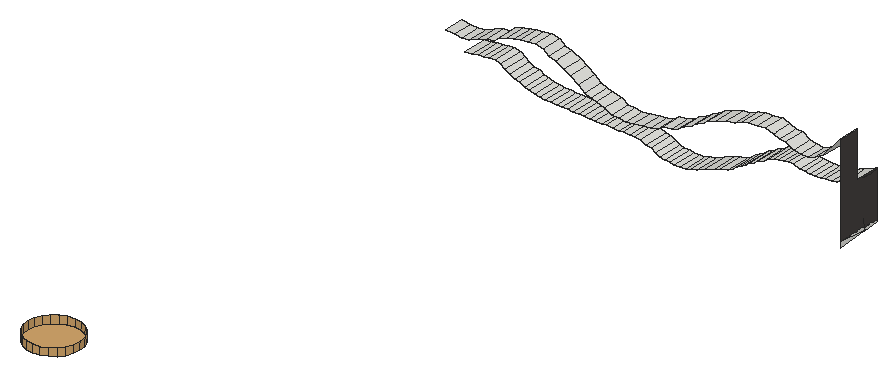
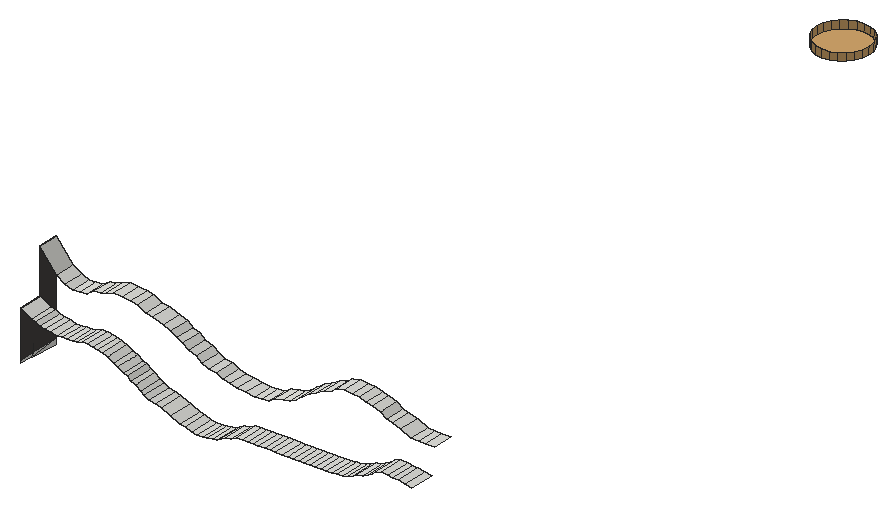
# SketchUp Ruby script. Lengths in inches.
U = 1.inch
M = Sketchup.active_model
def pt(a) = Geom::Point3d.new(a.map { |v| v * U })
def face(e, loops, mat)
  f = e.add_face(loops[0].map { |a| pt(a) })
  loops[1..].each { |l| e.add_face(l.map { |a| pt(a) }).erase! }
  f.material = f.back_material = mat if mat
  f
end
# faces: each face lists its corners as indices into pts; further lists are holes
def faces(e, pts, list, mat = nil) = list.each { |f| face(e, (f[0].is_a?(Array) ? f : [f]).map { |l| l.map { |i| pts[i] } }, mat) }
# xy, xz, yz: faces in a plane at the given z, y or x. An outline is a flat list of corners, or four numbers for a rectangle; further outlines are holes
def ring(l) = l.size == 4 ? [[l[0], l[1]], [l[2], l[1]], [l[2], l[3]], [l[0], l[3]]] : l.each_slice(2).to_a
def flat(e, list, mat, &to3) = list.each { |f| face(e, (f[0].is_a?(Array) ? f : [f]).map { |l| ring(l).map { |u, v| to3.(u, v) } }, mat) }
def xy(e, z, list, mat = nil) = flat(e, list, mat) { |x, y| [x, y, z] }
def xz(e, y, list, mat = nil) = flat(e, list, mat) { |x, z| [x, y, z] }
def yz(e, x, list, mat = nil) = flat(e, list, mat) { |y, z| [x, y, z] }
def lines(e, pts, list) = list.each { |a, b| e.add_line(pt(pts[a]), pt(pts[b])) }
# prism: a flat outline (further loops are holes) pulled along v
def prism(e, loops, v, mat = nil)
  f = face(e, loops, mat); d = Geom::Vector3d.new(v.map { |x| x * U })
  f.pushpull(f.normal.samedirection?(d) ? d.length : -d.length)
end
def box(e, o, s, mat = nil) = prism(e, [[o, [o[0] + s[0], o[1], o[2]], [o[0] + s[0], o[1] + s[1], o[2]], [o[0], o[1] + s[1], o[2]]]], [0, 0, s[2]], mat)
def at(x, y, z, deg = 0) = Geom::Transformation.translation(pt([x, y, z])) * Geom::Transformation.rotation(ORIGIN, Z_AXIS, deg.degrees)
def axes(o, x, y, z) = Geom::Transformation.new([*x, 0, *y, 0, *z, 0, *pt(o).to_a, 1])
def part(name) = M.definitions.add(name)
# library, detail: a bought-in or finely detailed component or shape, given as its bounding box
def library(name, o, s) = part(name).tap { |d| box(d.entities, o, s) }
def detail(e, o, s) = box(e.add_group.entities, o, s)
def put(e, d, t, mat = nil) = e.add_instance(d, t).tap { |i| i.material = mat if mat }
def group(e, t, mat = nil) = e.add_group.tap { |g| g.transformation = t; g.material = mat if mat }.entities
root = M.entities
M.materials.add("[Field Square Tile]").color = [211, 167, 108]
M.materials.add("[Granite Tile]1").color = [68, 65, 63]
xy(root,250.6875,[[2134.543,492.582,2133.831,492.675,2133.168,492.95,2132.598,493.387,2132.161,493.957,2131.886,494.62,2131.793,495.332,2131.886,496.043,2132.161,496.707,2132.598,497.276,2133.168,497.713,2133.831,497.988,2134.543,498.082,2135.254,497.988,2135.918,497.713,2136.487,497.276,2136.924,496.707,2137.199,496.043,2137.293,495.332,2137.199,494.62,2136.924,493.957,2136.487,493.387,2135.918,492.95,2135.254,492.675]],"[Field Square Tile]")
yz(root,2164.345,[[561.053,240.932,561.053,241.519,564.151,241.17],[564.185,241.167,564.151,241.17,564.184,241.173],[564.151,241.17,561.053,241.519,564.144,241.519,564.184,241.173],[564.184,241.173,564.144,241.519,565.74,241.519,565.74,241.293]])
yz(root,2164.345,[[561.053,241.519,561.053,251.165,563.178,251.165,563.178,246.426,565.74,246.426,565.74,241.519]],"[Granite Tile]1")
p = [[2144.767,563.178,241.17],[2144.767,565.74,241.17],[2145.237,565.74,241.121],[2145.237,563.178,241.121],[2145.843,565.74,241.09],[2145.843,563.178,241.09],
  [2146.41,565.74,241.138],[2146.41,563.178,241.138],[2147.05,565.74,241.346],[2147.05,563.178,241.346],[2143.769,563.178,241.332],[2143.769,565.74,241.332],
  [2144.237,565.74,241.243],[2144.237,563.178,241.243],[2143.35,563.178,241.566],[2143.35,565.74,241.566],[2147.641,565.74,241.456],[2147.641,563.178,241.456],
  [2148.576,565.74,241.847],[2148.576,563.178,241.847],[2142.844,563.178,241.837],[2142.844,565.74,241.837],[2142.271,563.178,241.967],[2142.271,565.74,241.967],
  [2149.581,565.74,242.229],[2149.581,563.178,242.229],[2141.69,563.178,242.199],[2141.69,565.74,242.199],[2141.064,563.178,242.277],[2141.064,565.74,242.277],
  [2150.142,565.74,242.424],[2150.142,563.178,242.424],[2135.217,563.178,242.35],[2135.217,565.74,242.35],[2135.799,565.74,242.342],[2135.799,563.178,242.342],
  [2136.381,565.74,242.334],[2136.381,563.178,242.334],[2136.963,565.74,242.326],[2136.963,563.178,242.326],[2137.683,565.74,242.317],[2137.683,563.178,242.317],
  [2138.153,565.74,242.312],[2138.153,563.178,242.312],[2138.794,565.74,242.304],[2138.794,563.178,242.304],[2139.458,565.74,242.296],[2139.458,563.178,242.296],
  [2139.91,565.74,242.291],[2139.91,563.178,242.291],[2140.548,565.74,242.283],[2140.548,563.178,242.283],[2131.735,563.178,242.466],[2131.735,565.74,242.466],
  [2132.311,565.74,242.428],[2132.311,563.178,242.428],[2132.89,565.74,242.403],[2132.89,563.178,242.403],[2133.47,565.74,242.385],[2133.47,563.178,242.385],
  [2134.052,565.74,242.371],[2134.052,563.178,242.371],[2134.634,565.74,242.36],[2134.634,563.178,242.36],[2150.86,565.74,242.605],[2150.86,563.178,242.605],
  [2130.607,563.178,242.599],[2130.607,565.74,242.599],[2131.167,565.74,242.518],[2131.167,563.178,242.518],[2130.054,563.178,242.75],[2130.054,565.74,242.75],
  [2151.373,565.74,242.907],[2151.373,563.178,242.907],[2129.566,563.178,242.921],[2129.566,565.74,242.921],[2129.075,563.178,243.216],[2129.075,565.74,243.216],
  [2151.745,565.74,243.144],[2151.745,563.178,243.144],[2152.294,565.74,243.516],[2152.294,563.178,243.516],[2128.527,563.178,243.332],[2128.527,565.74,243.332],
  [2127.982,563.178,243.589],[2127.982,565.74,243.589],[2152.768,565.74,243.711],[2152.768,563.178,243.711],[2127.501,563.178,243.88],[2127.501,565.74,243.88],
  [2153.099,565.74,244.02],[2153.099,563.178,244.02],[2127.124,563.178,244.194],[2127.124,565.74,244.194],[2123.336,563.178,243.992],[2123.336,565.74,243.992],
  [2124.039,565.74,244.076],[2124.039,563.178,244.076],[2153.543,565.74,244.206],[2153.543,563.178,244.206],[2124.738,565.74,244.207],[2124.738,563.178,244.207],
  [2125.323,565.74,244.266],[2125.323,563.178,244.266],[2126.527,563.178,244.387],[2126.527,565.74,244.387],[2154.132,565.74,244.569],[2154.132,563.178,244.569],
  [2125.864,565.74,244.296],[2125.864,563.178,244.296],[2154.602,565.74,244.757],[2154.602,563.178,244.757],[2155.219,565.74,245.125],[2155.219,563.178,245.125],
  [2140.415,561.053,245.064],[2140.415,563.178,245.064],[2141.125,563.178,244.949],[2141.125,561.053,244.949],[2141.839,563.178,244.867],[2141.839,561.053,244.867],
  [2142.745,563.178,245.007],[2142.745,561.053,245.007],[2143.689,563.178,245.121],[2143.689,561.053,245.121],[2139.702,561.053,245.459],[2139.702,563.178,245.459],
  [2144.454,563.178,245.254],[2144.454,561.053,245.254],[2155.723,565.74,245.32],[2155.723,563.178,245.32],[2159.424,563.178,245.272],[2159.424,565.74,245.272],
  [2159.982,565.74,245.235],[2159.982,563.178,245.235],[2160.536,565.74,245.216],[2160.536,563.178,245.216],[2161.101,565.74,245.34],[2161.101,563.178,245.34],
  [2145.206,563.178,245.41],[2145.206,561.053,245.41],[2156.205,565.74,245.411],[2156.205,563.178,245.411],[2157.771,563.178,245.552],[2157.771,565.74,245.552],
  [2158.379,565.74,245.346],[2158.379,563.178,245.346],[2158.873,565.74,245.309],[2158.873,563.178,245.309],[2161.733,565.74,245.423],[2161.733,563.178,245.423],
  [2145.84,563.178,245.775],[2145.84,561.053,245.775],[2156.753,565.74,245.481],[2156.753,563.178,245.481],[2162.311,565.74,245.516],[2162.311,563.178,245.516],
  [2138.827,561.053,245.671],[2138.827,563.178,245.671],[2157.235,565.74,245.59],[2157.235,563.178,245.59],[2162.691,565.74,245.763],[2162.691,563.178,245.763],
  [2138.152,561.053,245.834],[2138.152,563.178,245.834],[2137.564,561.053,246.129],[2137.564,563.178,246.129],[2146.636,563.178,245.88],[2146.636,561.053,245.88],
  [2163.16,565.74,245.896],[2163.16,563.178,245.896],[2147.349,563.178,246.16],[2147.349,561.053,246.16],[2164.345,565.74,246.426],[2164.345,563.178,246.426],
  [2136.933,561.053,246.633],[2136.933,563.178,246.633],[2147.946,563.178,246.573],[2147.946,561.053,246.573],[2136.119,561.053,247.185],[2136.119,563.178,247.185],
  [2148.736,563.178,246.902],[2148.736,561.053,246.902],[2123.942,561.053,246.79],[2123.942,563.178,246.79],[2124.721,563.178,246.747],[2124.721,561.053,246.747],
  [2125.468,563.178,246.831],[2125.468,561.053,246.831],[2122.988,561.053,246.838],[2122.988,563.178,246.838],[2126.51,563.178,247.251],[2126.51,561.053,247.251],
  [2149.338,563.178,247.347],[2149.338,561.053,247.347],[2135.407,561.053,247.553],[2135.407,563.178,247.553],[2127.384,563.178,247.546],[2127.384,561.053,247.546],
  [2150.012,563.178,247.615],[2150.012,561.053,247.615],[2128.046,563.178,247.657],[2128.046,561.053,247.657],[2134.516,561.053,248.059],[2134.516,563.178,248.059],
  [2150.599,563.178,248.057],[2150.599,561.053,248.057],[2128.679,563.178,248.162],[2128.679,561.053,248.162],[2133.825,561.053,248.257],[2133.825,563.178,248.257],
  [2151.364,563.178,248.322],[2151.364,561.053,248.322],[2129.473,563.178,248.408],[2129.473,561.053,248.408],[2160.161,561.053,248.295],[2160.161,563.178,248.295],
  [2160.87,563.178,248.218],[2160.87,561.053,248.218],[2161.687,563.178,248.558],[2161.687,561.053,248.558],[2133.294,561.053,248.687],[2133.294,563.178,248.687],
  [2152.475,563.178,248.655],[2152.475,561.053,248.655],[2159.45,561.053,248.42],[2159.45,563.178,248.42],[2130.172,563.178,248.521],[2130.172,561.053,248.521],
  [2158.653,561.053,248.895],[2158.653,563.178,248.895],[2130.866,563.178,248.723],[2130.866,561.053,248.723],[2162.622,563.178,249.022],[2162.622,561.053,249.022],
  [2131.565,563.178,248.801],[2131.565,561.053,248.801],[2132.462,561.053,248.851],[2132.462,563.178,248.851],[2153.248,563.178,248.795],[2153.248,561.053,248.795],
  [2154.111,563.178,249.194],[2154.111,561.053,249.194],[2157.949,561.053,248.962],[2157.949,563.178,248.962],[2157.31,561.053,249.206],[2157.31,563.178,249.206],
  [2164.345,563.178,251.165],[2164.345,561.053,251.165],[2154.784,563.178,249.323],[2154.784,561.053,249.323],[2156.565,561.053,249.478],[2156.565,563.178,249.478],
  [2155.707,563.178,249.406],[2155.707,561.053,249.406],[2134.543,492.582,251.5],[2133.831,492.675,251.5],[2133.831,492.675,250.6875],[2134.543,492.582,250.6875],
  [2135.254,492.675,251.5],[2135.254,492.675,250.6875],[2133.168,492.95,251.5],[2133.168,492.95,250.6875],[2135.918,492.95,251.5],[2135.918,492.95,250.6875],
  [2132.598,493.387,251.5],[2132.598,493.387,250.6875],[2136.487,493.387,251.5],[2136.487,493.387,250.6875],[2132.161,493.957,251.5],[2132.161,493.957,250.6875],
  [2136.924,493.957,251.5],[2136.924,493.957,250.6875],[2131.886,494.62,251.5],[2131.886,494.62,250.6875],[2137.199,494.62,251.5],[2137.199,494.62,250.6875],
  [2131.793,495.332,251.5],[2131.793,495.332,250.6875],[2137.293,495.332,251.5],[2137.293,495.332,250.6875],[2131.886,496.043,251.5],[2131.886,496.043,250.6875],
  [2137.199,496.043,251.5],[2137.199,496.043,250.6875],[2132.161,496.707,251.5],[2132.161,496.707,250.6875],[2136.924,496.707,251.5],[2136.924,496.707,250.6875],
  [2132.598,497.276,251.5],[2132.598,497.276,250.6875],[2136.487,497.276,251.5],[2136.487,497.276,250.6875],[2133.168,497.713,251.5],[2133.168,497.713,250.6875],
  [2135.918,497.713,251.5],[2135.918,497.713,250.6875],[2133.831,497.988,251.5],[2133.831,497.988,250.6875],[2135.254,497.988,251.5],[2135.254,497.988,250.6875],
  [2134.543,498.082,251.5],[2134.543,498.082,250.6875],[2164.345,564.963,246.171],[2164.345,563.948,246.265],[2164.345,564.144,241.519],[2164.345,564.042,242.384],
  [2164.345,565.74,246.273]]
faces(root,p,[[0,1,2,3],[3,2,4,5],[5,4,6,7],[7,6,8,9],[10,11,12,13],[13,12,1,0],[14,15,11,10],[9,8,16,17],
  [17,16,18,19],[20,21,15,14],[22,23,21,20],[19,18,24,25],[26,27,23,22],[28,29,27,26],[25,24,30,31],[32,33,34,35],
  [35,34,36,37],[37,36,38,39],[39,38,40,41],[41,40,42,43],[43,42,44,45],[45,44,46,47],[47,46,48,49],[49,48,50,51],
  [51,50,29,28],[52,53,54,55],[55,54,56,57],[57,56,58,59],[59,58,60,61],[61,60,62,63],[63,62,33,32],[31,30,64,65],
  [66,67,68,69],[69,68,53,52],[70,71,67,66],[65,64,72,73],[74,75,71,70],[76,77,75,74],[73,72,78,79],[79,78,80,81],
  [82,83,77,76],[84,85,83,82],[81,80,86,87],[88,89,85,84],[87,86,90,91],[92,93,89,88],[94,95,96,97],[91,90,98,99],
  [97,96,100,101],[101,100,102,103],[104,105,93,92],[99,98,106,107],[103,102,108,109],[109,108,105,104],[107,106,110,111],[111,110,112,113],
  [114,115,116,117],[117,116,118,119],[119,118,120,121],[121,120,122,123],[124,125,115,114],[123,122,126,127],[113,112,128,129],[130,131,132,133],
  [133,132,134,135],[135,134,136,137],[127,126,138,139],[129,128,140,141],[142,143,144,145],[145,144,146,147],[147,146,131,130],[137,136,148,149],
  [139,138,150,151],[141,140,152,153],[149,148,154,155],[156,157,125,124],[153,152,158,159],[155,154,160,161],[159,158,143,142],[162,163,157,156],
  [164,165,163,162],[151,150,166,167],[161,160,168,169],[167,166,170,171],[169,168,172,173],[174,175,165,164],[171,170,176,177],[178,179,175,174],
  [177,176,180,181],[182,183,184,185],[185,184,186,187],[188,189,183,182],[187,186,190,191],[181,180,192,193],[194,195,179,178],[191,190,196,197],
  [193,192,198,199],[197,196,200,201],[202,203,195,194],[199,198,204,205],[201,200,206,207],[208,209,203,202],[205,204,210,211],[207,206,212,213],
  [214,215,216,217],[217,216,218,219],[220,221,209,208],[211,210,222,223],[224,225,215,214],[213,212,226,227],[228,229,225,224],[227,226,230,231],
  [219,218,232,233],[231,230,234,235],[236,237,221,220],[223,222,238,239],[235,234,237,236],[239,238,240,241],[242,243,229,228],[244,245,243,242],
  [233,232,246,247],[241,240,248,249],[250,251,245,244],[249,248,252,253],[253,252,251,250]])
faces(root,p,[[254,255,256,257],[258,254,257,259],[255,260,261,256],[262,258,259,263],[260,264,265,261],[266,262,263,267],[264,268,269,265],[270,266,267,271],
  [268,272,273,269],[274,270,271,275],[272,276,277,273],[278,274,275,279],[276,280,281,277],[282,278,279,283],[280,284,285,281],[286,282,283,287],
  [284,288,289,285],[290,286,287,291],[288,292,293,289],[294,290,291,295],[292,296,297,293],[298,294,295,299],[296,300,301,297],[300,298,299,301]],"[Field Square Tile]")
lines(root,p,[[302,303],[304,305],[306,302]])
